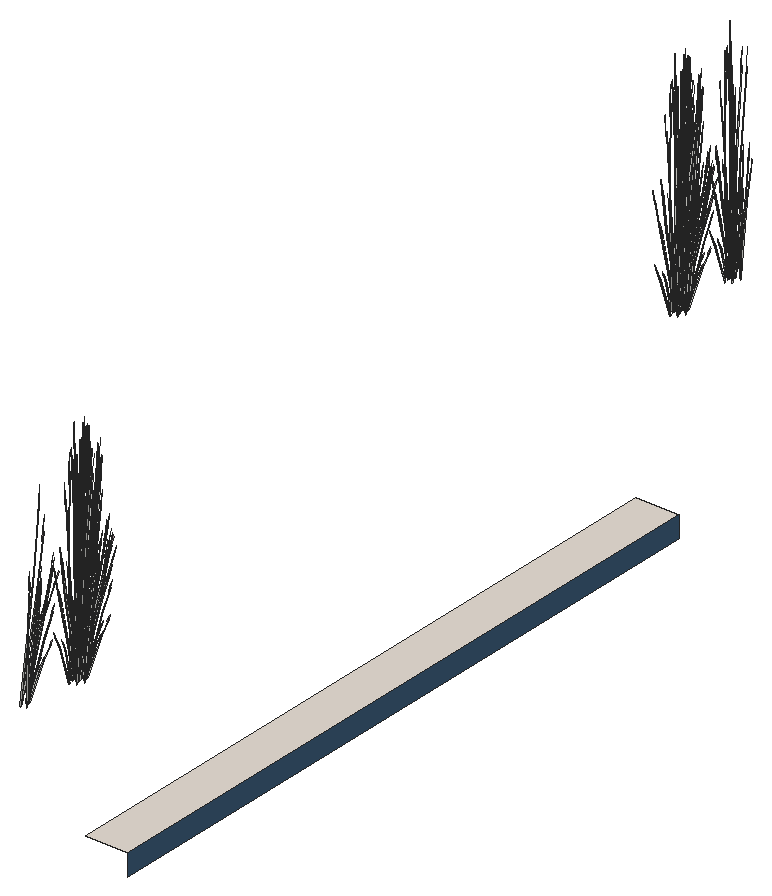
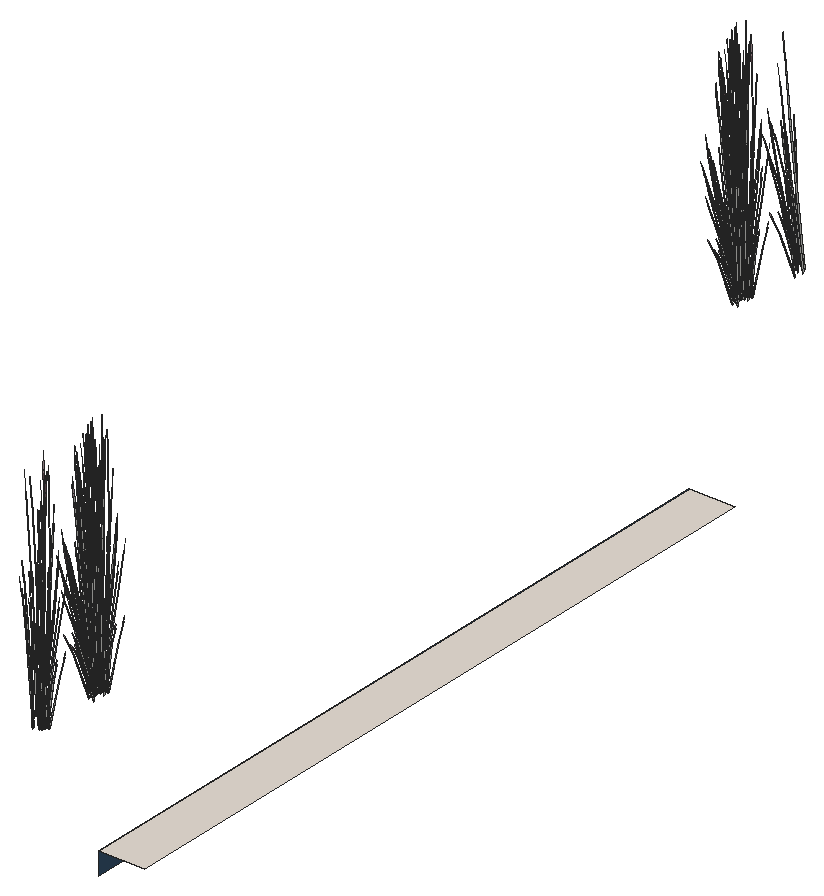
# SketchUp Ruby script. Lengths in inches.
U = 1.inch
M = Sketchup.active_model
def pt(a) = Geom::Point3d.new(a.map { |v| v * U })
def face(e, loops, mat)
  f = e.add_face(loops[0].map { |a| pt(a) })
  loops[1..].each { |l| e.add_face(l.map { |a| pt(a) }).erase! }
  f.material = f.back_material = mat if mat
  f
end
# faces: each face lists its corners as indices into pts; further lists are holes
def faces(e, pts, list, mat = nil) = list.each { |f| face(e, (f[0].is_a?(Array) ? f : [f]).map { |l| l.map { |i| pts[i] } }, mat) }
# xy, xz, yz: faces in a plane at the given z, y or x. An outline is a flat list of corners, or four numbers for a rectangle; further outlines are holes
def ring(l) = l.size == 4 ? [[l[0], l[1]], [l[2], l[1]], [l[2], l[3]], [l[0], l[3]]] : l.each_slice(2).to_a
def flat(e, list, mat, &to3) = list.each { |f| face(e, (f[0].is_a?(Array) ? f : [f]).map { |l| ring(l).map { |u, v| to3.(u, v) } }, mat) }
def xy(e, z, list, mat = nil) = flat(e, list, mat) { |x, y| [x, y, z] }
def xz(e, y, list, mat = nil) = flat(e, list, mat) { |x, z| [x, y, z] }
def yz(e, x, list, mat = nil) = flat(e, list, mat) { |y, z| [x, y, z] }
def lines(e, pts, list) = list.each { |a, b| e.add_line(pt(pts[a]), pt(pts[b])) }
# prism: a flat outline (further loops are holes) pulled along v
def prism(e, loops, v, mat = nil)
  f = face(e, loops, mat); d = Geom::Vector3d.new(v.map { |x| x * U })
  f.pushpull(f.normal.samedirection?(d) ? d.length : -d.length)
end
def box(e, o, s, mat = nil) = prism(e, [[o, [o[0] + s[0], o[1], o[2]], [o[0] + s[0], o[1] + s[1], o[2]], [o[0], o[1] + s[1], o[2]]]], [0, 0, s[2]], mat)
def at(x, y, z, deg = 0) = Geom::Transformation.translation(pt([x, y, z])) * Geom::Transformation.rotation(ORIGIN, Z_AXIS, deg.degrees)
def axes(o, x, y, z) = Geom::Transformation.new([*x, 0, *y, 0, *z, 0, *pt(o).to_a, 1])
def part(name) = M.definitions.add(name)
# library, detail: a bought-in or finely detailed component or shape, given as its bounding box
def library(name, o, s) = part(name).tap { |d| box(d.entities, o, s) }
def detail(e, o, s) = box(e.add_group.entities, o, s)
def put(e, d, t, mat = nil) = e.add_instance(d, t).tap { |i| i.material = mat if mat }
def group(e, t, mat = nil) = e.add_group.tap { |g| g.transformation = t; g.material = mat if mat }.entities
root = M.entities
M.materials.add("Carpet_04_1K").color = [56, 85, 112]
M.materials.add("LightPink_Translucent").color = [144, 107, 117]
M.materials["LightPink_Translucent"].alpha = 0.75
M.materials.add("Marble_01_1K").color = [230, 221, 211]
c1 = part("blade")
p = [[2.15,0.21,22],[0,0.17,0],[0.09,0.45,0],[2.18,0.31,22],[2.29,0.31,22],[0.38,0.45,0],
  [2.48,0.24,33],[2.49,0.24,33],[2.48,0.22,33]]
faces(c1.entities,p,[[0,1,2,3],[4,5,2,3],[6,3,4,7],[8,0,3,6]])
c2 = part("seeds")
p = [[0.3,-0.1,1.38],[-0.01,-0.03,1.59],[-0.01,-0.03,0.03],[0.14,-0.07,-0.07],[0.29,-0.03,3],[0.15,0.01,3.11]]
faces(c2.entities,p,[[0,1,2,3],[1,0,4,5]],"LightPink_Translucent")
c3 = part("blade with seeds")
put(c3.entities,c1,at(0,0,0))
put(c3.entities,c2,axes([2.4,0.25,30.99],[1.5799,-0.05474,1.17369],[-0.12525,1.92788,0.29478],[-0.07173,-0.02425,1.56792]))
xy(root,-42,[[398.57,316.3,410.57,509.26]],"Marble_01_1K")
yz(root,410.57,[[316.3,-48,509.26,-42]],"Carpet_04_1K")
put(root,c3,axes([400.96,292.9,1.98],[-0.22732,0.05597,1.41583],[-0.03618,-0.44548,0.08104],[0.15921,-0.06743,0.80566]))
put(root,c3,axes([401.37,292.51,2.26],[-0.21881,-0.29821,-0.06488],[0.23965,-0.27324,-0.29416],[0.0679,-0.01924,0.97024]))
put(root,c3,axes([400.54,292.9375,4.98],[0.31014,-0.20596,-0.71045],[0.17284,0.42397,0.08574],[0.14985,-0.04816,1.00501]))
put(root,c3,axes([401.2,292.61,1.49],[-0.01845,-0.0708,1.76342],[0.12793,-0.41416,-0.26939],[0.12905,-0.00596,0.30037]))
put(root,c3,axes([400.81,292.98,4.53],[0.29332,0.1301,-0.35414],[-0.08555,0.37955,0.4572],[0.11809,-0.0348,0.87481]))
put(root,c3,axes([400.29,291.34,2.02],[0.33032,0.23318,-0.49651],[-0.19744,0.41812,0],[0.07523,0.05311,1.57504]))
put(root,c3,axes([400.01,292.51,3.875],[-0.14639,0.01056,1.71376],[0.09712,-0.45778,0.13857],[0.20862,0.02831,0.73262]))
put(root,c3,axes([399.81,292.23,2.06],[0.36714,0.07646,-0.62353],[-0.07747,0.47163,-0.16365],[0.10956,0.05715,1.37633]))
put(root,c3,axes([401.43,293.06,2.77],[-0.21807,0.07699,1.1486],[0.10265,-0.31819,0.84392],[0.11568,0.02177,0.25299]))
put(root,c3,axes([401.05,294.04,3.93],[-0.06755,-0.39203,-0.03492],[0.31928,-0.09013,-0.15832],[0.06667,0.02485,0.52218]))
put(root,c3,axes([401.02,293.57,2.59],[-0.085,-0.1147,1.43002],[0.1106,-0.37943,-0.30754],[0.17198,0.0514,0.61141]))
put(root,c3,axes([400.24,293.8,4.98],[0.35281,0.01123,-0.71045],[-0.0237,0.47284,0.08574],[0.14947,0.0499,1.00501]))
put(root,c3,axes([400.45,293.99,4.53],[0.20082,0.29199,-0.35414],[-0.2293,0.2764,0.4572],[0.1165,0.04206,0.87481]))
put(root,c3,axes([399.73,293.24,3.875],[-0.1311,-0.08035,1.71376],[0.27131,-0.33708,0.13857],[0.16909,0.15206,0.73262]))
put(root,c3,axes([400.27,294.66,1.49],[0.02571,-0.06733,1.76342],[0.32373,-0.19829,-0.26939],[0.09815,0.10263,0.30037]))
put(root,c3,axes([399.77,294.34,4.68],[0.34827,-0.11086,-0.51099],[0.06092,0.41983,-0.3958],[0.09354,0.12031,0.97773]))
put(root,c3,axes([402.72,307.125,2.59],[-0.10032,0.0944,1.43002],[-0.30046,-0.16522,-0.30754],[0.05569,-0.20547,0.61141]))
put(root,c3,axes([401.98,306.61,1.49],[-0.0592,0.0168,1.76342],[-0.32738,-0.18913,-0.26939],[0.00549,-0.15776,0.30037]))
put(root,c3,axes([402.97,307.83,4.98],[0.00918,-0.43138,-0.71045],[0.38672,0.02897,0.08574],[0.04081,-0.18275,1.00501]))
put(root,c3,axes([402.3,307.13,4.53],[0.1064,-0.35863,-0.35414],[0.31043,0.1046,0.4572],[-0.02846,-0.14439,0.87481]))
put(root,c3,axes([402.53,307.61,3.875],[-0.06572,0.16029,1.71376],[-0.27569,-0.33172,0.13857],[0.12437,-0.20675,0.73262]))
put(root,c3,axes([402.35,306.375,2.77],[0.04528,0.27194,1.1486],[-0.25117,-0.15062,0.84392],[0.02703,-0.13924,0.25299]))
put(root,c3,axes([402.89,307.68,4.68],[-0.25266,-0.31335,-0.51099],[0.2669,-0.27442,-0.3958],[0.03844,-0.15921,0.97773]))
put(root,c3,axes([403.13,307.57,4.53],[0.23881,-0.24554,-0.35414],[0.22606,0.28036,0.4572],[0.0344,-0.14245,0.87481]))
put(root,c3,axes([403.43,307.42,1.49],[-0.05283,-0.03674,1.76342],[-0.13569,-0.41045,-0.26939],[0.09154,-0.11138,0.30037]))
put(root,c3,axes([403.42,308.57,4.98],[0.18436,-0.36797,-0.71045],[0.32306,0.26151,0.08574],[0.11008,-0.13332,1.00501]))
put(root,c3,axes([401.43,307.5,2.375],[-0.22066,-0.46731,0],[0.36918,-0.26061,-0.51607],[0.08408,-0.05936,1.63711]))
put(root,c3,axes([403.41,308.4,4.68],[-0.09067,-0.42583,-0.51099],[0.34336,-0.07449,-0.3958],[0.0984,-0.11438,0.97773]))
put(root,c3,axes([401.73,307.43,2.02],[0.33032,-0.23318,-0.49651],[0.19744,0.41812,0],[0.07523,-0.05311,1.57504]))
put(root,c3,axes([403.69,308.24,2.59],[-0.12609,-0.01381,1.43002],[-0.12917,-0.37055,-0.30754],[0.1549,-0.10482,0.61141]))
put(root,c3,axes([402.12,308.39,2.06],[0.23773,-0.35053,-0.62353],[0.29532,0.31785,-0.16365],[0.09526,-0.08744,1.37633]))
put(root,c3,axes([403.84,307.56,2.77],[-0.11756,0.2374,1.1486],[-0.10105,-0.31895,0.84392],[0.09709,-0.07992,0.25299]))
put(root,c3,axes([403.67,308.45,4.53],[0.30722,-0.06665,-0.35414],[0.08112,0.381,0.4572],[0.08804,-0.10234,0.87481]))
put(root,c3,axes([401.71,309,2.21],[0.17124,-0.42022,-0.44739],[0.35581,0.20224,0.21531],[0,-0.09687,1.43643]))
put(root,c3,axes([401.86,308.79,2.67],[-0.04113,-0.53214,-0.29095],[0.42835,-0.03218,-0.50002],[0.07543,-0.07088,1.59708]))
put(root,c3,axes([401.81,307.62,2.03],[0.32928,0.11539,-0.30978],[-0.08291,0.40636,0.30978],[0.06638,-0.04686,1.38974]))
put(root,c3,axes([401.92,309.21,2.43],[0.39767,0.22603,0.24065],[-0.19139,0.46966,0.50002],[0,-0.10827,1.60543]))
put(root,c3,axes([401.79,308.9,2.72],[-0.38326,0.02879,0.44739],[-0.03466,-0.47788,-0.21531],[0.06861,-0.04843,1.43643]))
put(root,c3,axes([403.57,309.35,4.68],[0.09562,-0.42421,-0.51099],[0.32782,0.1454,-0.3958],[0.13199,-0.0389,0.97773]))
put(root,c3,axes([403.06,307.62,2.375],[0.22066,-0.46731,0],[0.36918,0.26061,-0.51607],[0.08408,0.05936,1.63711]))
put(root,c3,axes([401.78,309.07,2.36],[0.15345,0.52148,0.45755],[-0.43845,0.18134,0.17955],[0.00536,-0.09582,1.58856]))
put(root,c3,axes([403.92,309.47,1.98],[-0.22732,0.05597,1.41583],[-0.03618,-0.44548,0.08104],[0.15921,-0.06743,0.80566]))
put(root,c3,axes([404.34,309.07,2.26],[-0.21881,-0.29821,-0.06488],[0.23965,-0.27324,-0.29416],[0.0679,-0.01924,0.97024]))
put(root,c3,axes([402.33,309.11,2.21],[0,-0.53961,0],[0.44133,0,0],[0,0,1.79456]))
put(root,c3,axes([402.87,307.87,2.48],[-0.33032,-0.23318,0.49651],[0.19744,-0.41812,0],[0.07523,0.05311,1.57504]))
put(root,c3,axes([403.51,309.5,4.98],[0.31014,-0.20596,-0.71045],[0.17284,0.42397,0.08574],[0.14985,-0.04816,1.00501]))
put(root,c3,axes([402.12,308.77,2.36],[-0.29264,0.42323,0.45755],[-0.34767,-0.3736,0.17955],[0.07055,-0.04224,1.58856]))
put(root,c3,axes([401.61,308.08,2.47],[-0.10196,0.46348,0.17642],[-0.3731,-0.13116,0.35086],[0.06445,-0.00226,1.60407]))
put(root,c3,axes([401.46,308.45,1.59],[-0.3474,0.18671,1.28929],[-0.11057,-0.53572,0.50096],[0.21332,0.00891,1.46642]))
put(root,c3,axes([402.39,308.59,2.62],[0.06809,-0.4162,0.1448],[0.33266,0.07225,-0.41347],[0.06054,0.04274,1.26744]))
put(root,c3,axes([404.17,309.18,1.49],[-0.01845,-0.0708,1.76342],[0.12793,-0.41416,-0.26939],[0.12905,-0.00596,0.30037]))
put(root,c3,axes([402.25,308.7,2.72],[-0.21202,-0.39143,0.44739],[0.32115,-0.27564,-0.21531],[0.06861,0.04843,1.43643]))
put(root,c3,axes([402.36,308.73,2.67],[0.35635,-0.30962,-0.29095],[0.23697,0.43749,-0.50002],[0.08792,0.04443,1.59708]))
put(root,c3,axes([403.78,309.54,4.53],[0.29332,0.1301,-0.35414],[-0.08555,0.37955,0.4572],[0.11809,-0.0348,0.87481]))
put(root,c3,axes([403.26,307.9,2.02],[0.33032,0.23318,-0.49651],[-0.19744,0.41812,0],[0.07523,0.05311,1.57504]))
put(root,c3,axes([402.63,309.23,2.21],[0.39487,0,0],[0,0.48281,0],[0,0,1.78407]))
put(root,c3,axes([402.74,308.1,2.47],[-0.37926,0.12378,0.17642],[-0.09365,-0.46065,0.35086],[0.03382,0.06712,1.60407]))
put(root,c3,axes([402.98,309.07,3.875],[-0.14639,0.01056,1.71376],[0.09712,-0.45778,0.13857],[0.20862,0.02831,0.73262]))
put(root,c3,axes([403.17,308.08,2.03],[0.08291,0.40636,-0.30978],[-0.32928,0.11539,0.30978],[0.06638,0.04686,1.38974]))
put(root,c3,axes([402.5,308.99,2.38],[-0.44609,-0.09826,0.49198],[0.09078,-0.55493,0.19306],[0.06519,0.05359,1.70813]))
put(root,c3,axes([402.15,310.36,2.2],[-0.11516,-0.40207,0],[0.32884,-0.1408,0],[0,0,1.54371]))
put(root,c3,axes([402.58,310.3,2.18],[0.37054,-0.15823,-0.19198],[0.1302,0.45581,0.00008],[0.0409,-0.01749,1.73897]))
put(root,c3,axes([402.62,309.44,2.21],[0.24637,0.30123,0],[-0.24637,0.30123,0],[0,0,1.69266]))
put(root,c3,axes([403.29,309.31,2.47],[-0.2773,-0.3397,0.17642],[0.27945,-0.32949,0.35086],[-0.03063,0.06937,1.60407]))
put(root,c3,axes([402.78,308.8,2.06],[0.36714,0.07646,-0.62353],[-0.07747,0.47163,-0.16365],[0.10956,0.05715,1.37633]))
put(root,c3,axes([404.4,309.62,2.77],[-0.21807,0.07699,1.1486],[0.10265,-0.31819,0.84392],[0.11568,0.02177,0.25299]))
put(root,c3,axes([402.62,309.09,2.72],[0.17124,-0.42022,0.44739],[0.35581,0.20224,-0.21531],[0,0.09687,1.43643]))
put(root,c3,axes([402.55,309.33,2.29],[0,0.53934,-0.05637],[-0.44133,0,0],[0,0.01695,1.79368]))
put(root,c3,axes([402.58,308.95,2.21],[0.21202,0.39143,-0.44739],[-0.32115,0.27564,0.21531],[0.06861,0.04843,1.43643]))
put(root,c3,axes([404.02,310.6,3.93],[-0.06755,-0.39203,-0.03492],[0.31928,-0.09013,-0.15832],[0.06667,0.02485,0.52218]))
put(root,c3,axes([403.52,309.32,2.48],[0,-0.46636,0.49651],[0.39487,0,0],[0,0.10622,1.57504]))
put(root,c3,axes([402.77,309.18,2.62],[0.32884,-0.136,0.1448],[0.11516,0.38837,-0.41347],[0,0.08547,1.26744]))
put(root,c3,axes([403.99,310.13,2.59],[-0.085,-0.1147,1.43002],[0.1106,-0.37943,-0.30754],[0.17198,0.0514,0.61141]))
put(root,c3,axes([402.47,310.55,2.2],[0.35581,0.20937,0],[-0.17124,0.43505,0],[0,0,1.74954]))
put(root,c3,axes([403.21,310.36,4.98],[0.35281,0.01123,-0.71045],[-0.0237,0.47284,0.08574],[0.14947,0.0499,1.00501]))
put(root,c3,axes([402.8125,310.74,2.48],[0.33032,-0.23318,0.49651],[0.19744,0.41812,0],[-0.07523,0.05311,1.57504]))
put(root,c3,axes([402.34,310.37,2.29],[0.15345,0.53576,-0.06012],[-0.43845,0.18773,0],[0.00536,0.01871,1.72173]))
put(root,c3,axes([403.78,309.4,2.375],[0.44133,0,0],[0,0.52122,-0.51607],[0,0.11871,1.63711]))
put(root,c3,axes([403.61,309.67,2.2],[-0.44111,-0.00373,-0.04976],[0,-0.52122,0.49943],[-0.01386,0.11865,1.58352]))
put(root,c3,axes([402.65,309.22,2.67],[0.39748,0.22252,-0.29095],[-0.19139,0.46966,-0.50002],[0.01249,0.11531,1.59708]))
put(root,c3,axes([403.42,310.56,4.53],[0.20082,0.29199,-0.35414],[-0.2293,0.2764,0.4572],[0.1165,0.04206,0.87481]))
put(root,c3,axes([403.52,309.74,2.03],[-0.24637,0.29097,-0.30978],[-0.24637,-0.29097,0.30978],[0,0.09372,1.38974]))
put(root,c3,axes([402.61,309.5625,2.21],[-0.17124,0.42022,-0.44739],[-0.35581,-0.20224,0.21531],[0,0.09687,1.43643]))
put(root,c3,axes([402.62,310.77,2.33],[0.44186,0.15158,0.30756],[-0.11054,0.54181,-0.36492],[-0.07313,0.06781,1.64885]))
put(root,c3,axes([403.6875,309.75,2.02],[0,0.46636,-0.49651],[-0.39487,0,0],[0,0.10622,1.57504]))
put(root,c3,axes([402.7,309.81,3.875],[-0.1311,-0.08035,1.71376],[0.27131,-0.33708,0.13857],[0.16909,0.15206,0.73262]))
put(root,c3,axes([403.18,310.72,2.77],[-0.19872,-0.13409,1.1486],[0.2566,-0.13625,0.84392],[0.06921,0.11541,0.25299]))
put(root,c3,axes([403.24,311.22,1.49],[0.02571,-0.06733,1.76342],[0.32373,-0.19829,-0.26939],[0.09815,0.10263,0.30037]))
put(root,c3,axes([402.8125,309.69,2.09],[0.12941,0.42699,-0.69212],[-0.37279,0.15378,-0.18165],[0.0143,0.14459,1.52773]))
put(root,c3,axes([402.74,310.91,4.68],[0.34827,-0.11086,-0.51099],[0.06092,0.41983,-0.3958],[0.09354,0.12031,0.97773]))
put(root,c3,axes([403.22,311.33,2.67],[-0.22633,-0.01463,1.0506],[0.14947,-0.31064,0.58006],[0.08941,0.11036,0.8241]))
put(root,c3,axes([402.48,310.58,2.59],[0.00623,-0.15459,1.43002],[0.29764,-0.17268,-0.30754],[0.09188,0.18503,0.61141]))
put(root,c3,axes([401.73,311.21,1.49],[0.05712,-0.02538,1.76342],[0.34359,0.13968,-0.26939],[0.01005,0.15742,0.30037]))
put(root,c3,axes([401.96,311.1,4.68],[0.34695,0.11691,-0.51099],[-0.11892,0.40083,-0.3958],[0.03181,0.16138,0.97773]))
put(root,c3,axes([402.16,310.27,3.875],[-0.08068,-0.14973,1.71376],[0.3728,-0.12606,0.13857],[0.08426,0.23506,0.73262]))
put(root,c3,axes([401.8,311.35,4.53],[-0.1064,0.35863,-0.35414],[-0.31043,-0.1046,0.4572],[0.02846,0.14439,0.87481]))
put(root,c3,axes([401.84,311.03,4.98],[0.16845,0.3792,-0.71045],[-0.34676,0.21133,0.08574],[0.03939,0.18322,1.00501]))
put(root,c3,axes([402.72,517.5625,2.59],[-0.10032,0.0944,1.43002],[-0.30046,-0.16522,-0.30754],[0.05569,-0.20547,0.61141]))
put(root,c3,axes([401.98,517.05,1.49],[-0.0592,0.0168,1.76342],[-0.32738,-0.18913,-0.26939],[0.00549,-0.15776,0.30037]))
put(root,c3,axes([402.97,518.26,4.98],[0.00918,-0.43138,-0.71045],[0.38672,0.02897,0.08574],[0.04081,-0.18275,1.00501]))
put(root,c3,axes([402.3,517.57,4.53],[0.1064,-0.35863,-0.35414],[0.31043,0.1046,0.4572],[-0.02846,-0.14439,0.87481]))
put(root,c3,axes([402.53,518.04,3.875],[-0.06572,0.16029,1.71376],[-0.27569,-0.33172,0.13857],[0.12437,-0.20675,0.73262]))
put(root,c3,axes([402.35,516.81,2.77],[0.04528,0.27194,1.1486],[-0.25117,-0.15062,0.84392],[0.02703,-0.13924,0.25299]))
put(root,c3,axes([402.89,518.12,4.68],[-0.25266,-0.31335,-0.51099],[0.2669,-0.27442,-0.3958],[0.03844,-0.15921,0.97773]))
put(root,c3,axes([403.13,518,4.53],[0.23881,-0.24554,-0.35414],[0.22606,0.28036,0.4572],[0.0344,-0.14245,0.87481]))
put(root,c3,axes([403.43,517.85,1.49],[-0.05283,-0.03674,1.76342],[-0.13569,-0.41045,-0.26939],[0.09154,-0.11138,0.30037]))
put(root,c3,axes([403.42,519.01,4.98],[0.18436,-0.36797,-0.71045],[0.32306,0.26151,0.08574],[0.11008,-0.13332,1.00501]))
put(root,c3,axes([401.43,517.9375,2.375],[-0.22066,-0.46731,0],[0.36918,-0.26061,-0.51607],[0.08408,-0.05936,1.63711]))
put(root,c3,axes([403.41,518.84,4.68],[-0.09067,-0.42583,-0.51099],[0.34336,-0.07449,-0.3958],[0.0984,-0.11438,0.97773]))
put(root,c3,axes([401.73,517.87,2.02],[0.33032,-0.23318,-0.49651],[0.19744,0.41812,0],[0.07523,-0.05311,1.57504]))
put(root,c3,axes([403.69,518.67,2.59],[-0.12609,-0.01381,1.43002],[-0.12917,-0.37055,-0.30754],[0.1549,-0.10482,0.61141]))
put(root,c3,axes([402.12,518.82,2.06],[0.23773,-0.35053,-0.62353],[0.29532,0.31785,-0.16365],[0.09526,-0.08744,1.37633]))
put(root,c3,axes([403.84,517.99,2.77],[-0.11756,0.2374,1.1486],[-0.10105,-0.31895,0.84392],[0.09709,-0.07992,0.25299]))
put(root,c3,axes([403.67,518.88,4.53],[0.30722,-0.06665,-0.35414],[0.08112,0.381,0.4572],[0.08804,-0.10234,0.87481]))
put(root,c3,axes([401.71,519.4375,2.21],[0.17124,-0.42022,-0.44739],[0.35581,0.20224,0.21531],[0,-0.09687,1.43643]))
put(root,c3,axes([401.86,519.23,2.67],[-0.04113,-0.53214,-0.29095],[0.42835,-0.03218,-0.50002],[0.07543,-0.07088,1.59708]))
put(root,c3,axes([401.81,518.05,2.03],[0.32928,0.11539,-0.30978],[-0.08291,0.40636,0.30978],[0.06638,-0.04686,1.38974]))
put(root,c3,axes([401.92,519.65,2.43],[0.39767,0.22603,0.24065],[-0.19139,0.46966,0.50002],[0,-0.10827,1.60543]))
put(root,c3,axes([401.79,519.33,2.72],[-0.38326,0.02879,0.44739],[-0.03466,-0.47788,-0.21531],[0.06861,-0.04843,1.43643]))
put(root,c3,axes([403.57,519.78,4.68],[0.09562,-0.42421,-0.51099],[0.32782,0.1454,-0.3958],[0.13199,-0.0389,0.97773]))
put(root,c3,axes([403.06,518.06,2.375],[0.22066,-0.46731,0],[0.36918,0.26061,-0.51607],[0.08408,0.05936,1.63711]))
put(root,c3,axes([401.78,519.5,2.36],[0.15345,0.52148,0.45755],[-0.43845,0.18134,0.17955],[0.00536,-0.09582,1.58856]))
put(root,c3,axes([403.92,519.9,1.98],[-0.22732,0.05597,1.41583],[-0.03618,-0.44548,0.08104],[0.15921,-0.06743,0.80566]))
put(root,c3,axes([404.34,519.51,2.26],[-0.21881,-0.29821,-0.06488],[0.23965,-0.27324,-0.29416],[0.0679,-0.01924,0.97024]))
put(root,c3,axes([402.33,519.55,2.21],[0,-0.53961,0],[0.44133,0,0],[0,0,1.79456]))
put(root,c3,axes([402.87,518.3,2.48],[-0.33032,-0.23318,0.49651],[0.19744,-0.41812,0],[0.07523,0.05311,1.57504]))
put(root,c3,axes([403.51,519.9375,4.98],[0.31014,-0.20596,-0.71045],[0.17284,0.42397,0.08574],[0.14985,-0.04816,1.00501]))
put(root,c3,axes([402.12,519.21,2.36],[-0.29264,0.42323,0.45755],[-0.34767,-0.3736,0.17955],[0.07055,-0.04224,1.58856]))
put(root,c3,axes([401.61,518.51,2.47],[-0.10196,0.46348,0.17642],[-0.3731,-0.13116,0.35086],[0.06445,-0.00226,1.60407]))
put(root,c3,axes([401.46,518.89,1.59],[-0.3474,0.18671,1.28929],[-0.11057,-0.53572,0.50096],[0.21332,0.00891,1.46642]))
put(root,c3,axes([402.39,519.03,2.62],[0.06809,-0.4162,0.1448],[0.33266,0.07225,-0.41347],[0.06054,0.04274,1.26744]))
put(root,c3,axes([404.17,519.61,1.49],[-0.01845,-0.0708,1.76342],[0.12793,-0.41416,-0.26939],[0.12905,-0.00596,0.30037]))
put(root,c3,axes([402.25,519.14,2.72],[-0.21202,-0.39143,0.44739],[0.32115,-0.27564,-0.21531],[0.06861,0.04843,1.43643]))
put(root,c3,axes([402.36,519.16,2.67],[0.35635,-0.30962,-0.29095],[0.23697,0.43749,-0.50002],[0.08792,0.04443,1.59708]))
put(root,c3,axes([403.78,519.98,4.53],[0.29332,0.1301,-0.35414],[-0.08555,0.37955,0.4572],[0.11809,-0.0348,0.87481]))
put(root,c3,axes([403.26,518.34,2.02],[0.33032,0.23318,-0.49651],[-0.19744,0.41812,0],[0.07523,0.05311,1.57504]))
put(root,c3,axes([402.63,519.67,2.21],[0.39487,0,0],[0,0.48281,0],[0,0,1.78407]))
put(root,c3,axes([402.74,518.54,2.47],[-0.37926,0.12378,0.17642],[-0.09365,-0.46065,0.35086],[0.03382,0.06712,1.60407]))
put(root,c3,axes([402.98,519.51,3.875],[-0.14639,0.01056,1.71376],[0.09712,-0.45778,0.13857],[0.20862,0.02831,0.73262]))
put(root,c3,axes([403.17,518.51,2.03],[0.08291,0.40636,-0.30978],[-0.32928,0.11539,0.30978],[0.06638,0.04686,1.38974]))
put(root,c3,axes([402.5,519.42,2.38],[-0.44609,-0.09826,0.49198],[0.09078,-0.55493,0.19306],[0.06519,0.05359,1.70813]))
put(root,c3,axes([402.15,520.79,2.2],[-0.11516,-0.40207,0],[0.32884,-0.1408,0],[0,0,1.54371]))
put(root,c3,axes([402.58,520.74,2.18],[0.37054,-0.15823,-0.19198],[0.1302,0.45581,0.00008],[0.0409,-0.01749,1.73897]))
put(root,c3,axes([402.62,519.875,2.21],[0.24637,0.30123,0],[-0.24637,0.30123,0],[0,0,1.69266]))
put(root,c3,axes([403.29,519.74,2.47],[-0.2773,-0.3397,0.17642],[0.27945,-0.32949,0.35086],[-0.03063,0.06937,1.60407]))
put(root,c3,axes([402.78,519.23,2.06],[0.36714,0.07646,-0.62353],[-0.07747,0.47163,-0.16365],[0.10956,0.05715,1.37633]))
put(root,c3,axes([404.4,520.06,2.77],[-0.21807,0.07699,1.1486],[0.10265,-0.31819,0.84392],[0.11568,0.02177,0.25299]))
put(root,c3,axes([402.62,519.52,2.72],[0.17124,-0.42022,0.44739],[0.35581,0.20224,-0.21531],[0,0.09687,1.43643]))
put(root,c3,axes([402.55,519.76,2.29],[0,0.53934,-0.05637],[-0.44133,0,0],[0,0.01695,1.79368]))
put(root,c3,axes([402.58,519.38,2.21],[0.21202,0.39143,-0.44739],[-0.32115,0.27564,0.21531],[0.06861,0.04843,1.43643]))
put(root,c3,axes([404.02,521.04,3.93],[-0.06755,-0.39203,-0.03492],[0.31928,-0.09013,-0.15832],[0.06667,0.02485,0.52218]))
put(root,c3,axes([403.52,519.76,2.48],[0,-0.46636,0.49651],[0.39487,0,0],[0,0.10622,1.57504]))
put(root,c3,axes([402.77,519.62,2.62],[0.32884,-0.136,0.1448],[0.11516,0.38837,-0.41347],[0,0.08547,1.26744]))
put(root,c3,axes([403.99,520.57,2.59],[-0.085,-0.1147,1.43002],[0.1106,-0.37943,-0.30754],[0.17198,0.0514,0.61141]))
put(root,c3,axes([402.47,520.98,2.2],[0.35581,0.20937,0],[-0.17124,0.43505,0],[0,0,1.74954]))
put(root,c3,axes([403.21,520.8,4.98],[0.35281,0.01123,-0.71045],[-0.0237,0.47284,0.08574],[0.14947,0.0499,1.00501]))
put(root,c3,axes([402.8125,521.18,2.48],[0.33032,-0.23318,0.49651],[0.19744,0.41812,0],[-0.07523,0.05311,1.57504]))
put(root,c3,axes([402.34,520.81,2.29],[0.15345,0.53576,-0.06012],[-0.43845,0.18773,0],[0.00536,0.01871,1.72173]))
put(root,c3,axes([403.78,519.84,2.375],[0.44133,0,0],[0,0.52122,-0.51607],[0,0.11871,1.63711]))
put(root,c3,axes([403.61,520.1,2.2],[-0.44111,-0.00373,-0.04976],[0,-0.52122,0.49943],[-0.01386,0.11865,1.58352]))
put(root,c3,axes([402.65,519.65,2.67],[0.39748,0.22252,-0.29095],[-0.19139,0.46966,-0.50002],[0.01249,0.11531,1.59708]))
put(root,c3,axes([403.42,520.99,4.53],[0.20082,0.29199,-0.35414],[-0.2293,0.2764,0.4572],[0.1165,0.04206,0.87481]))
put(root,c3,axes([403.52,520.18,2.03],[-0.24637,0.29097,-0.30978],[-0.24637,-0.29097,0.30978],[0,0.09372,1.38974]))
put(root,c3,axes([402.61,520,2.21],[-0.17124,0.42022,-0.44739],[-0.35581,-0.20224,0.21531],[0,0.09687,1.43643]))
put(root,c3,axes([402.62,521.21,2.33],[0.44186,0.15158,0.30756],[-0.11054,0.54181,-0.36492],[-0.07313,0.06781,1.64885]))
put(root,c3,axes([403.6875,520.19,2.02],[0,0.46636,-0.49651],[-0.39487,0,0],[0,0.10622,1.57504]))
put(root,c3,axes([402.7,520.24,3.875],[-0.1311,-0.08035,1.71376],[0.27131,-0.33708,0.13857],[0.16909,0.15206,0.73262]))
put(root,c3,axes([403.18,521.16,2.77],[-0.19872,-0.13409,1.1486],[0.2566,-0.13625,0.84392],[0.06921,0.11541,0.25299]))
put(root,c3,axes([403.24,521.66,1.49],[0.02571,-0.06733,1.76342],[0.32373,-0.19829,-0.26939],[0.09815,0.10263,0.30037]))
put(root,c3,axes([402.8125,520.125,2.09],[0.12941,0.42699,-0.69212],[-0.37279,0.15378,-0.18165],[0.0143,0.14459,1.52773]))
put(root,c3,axes([402.74,521.34,4.68],[0.34827,-0.11086,-0.51099],[0.06092,0.41983,-0.3958],[0.09354,0.12031,0.97773]))
put(root,c3,axes([403.22,521.77,2.67],[-0.22633,-0.01463,1.0506],[0.14947,-0.31064,0.58006],[0.08941,0.11036,0.8241]))
put(root,c3,axes([402.48,521.01,2.59],[0.00623,-0.15459,1.43002],[0.29764,-0.17268,-0.30754],[0.09188,0.18503,0.61141]))
put(root,c3,axes([401.73,521.64,1.49],[0.05712,-0.02538,1.76342],[0.34359,0.13968,-0.26939],[0.01005,0.15742,0.30037]))
put(root,c3,axes([401.96,521.54,4.68],[0.34695,0.11691,-0.51099],[-0.11892,0.40083,-0.3958],[0.03181,0.16138,0.97773]))
put(root,c3,axes([402.16,520.71,3.875],[-0.08068,-0.14973,1.71376],[0.3728,-0.12606,0.13857],[0.08426,0.23506,0.73262]))
put(root,c3,axes([401.8,521.78,4.53],[-0.1064,0.35863,-0.35414],[-0.31043,-0.1046,0.4572],[0.02846,0.14439,0.87481]))
put(root,c3,axes([401.84,521.46,4.98],[0.16845,0.3792,-0.71045],[-0.34676,0.21133,0.08574],[0.03939,0.18322,1.00501]))
put(root,c3,axes([402.72,536.79,2.59],[-0.10032,0.0944,1.43002],[-0.30046,-0.16522,-0.30754],[0.05569,-0.20547,0.61141]))
put(root,c3,axes([401.98,536.28,1.49],[-0.0592,0.0168,1.76342],[-0.32738,-0.18913,-0.26939],[0.00549,-0.15776,0.30037]))
put(root,c3,axes([402.97,537.49,4.98],[0.00918,-0.43138,-0.71045],[0.38672,0.02897,0.08574],[0.04081,-0.18275,1.00501]))
put(root,c3,axes([402.3,536.8,4.53],[0.1064,-0.35863,-0.35414],[0.31043,0.1046,0.4572],[-0.02846,-0.14439,0.87481]))
put(root,c3,axes([402.53,537.27,3.875],[-0.06572,0.16029,1.71376],[-0.27569,-0.33172,0.13857],[0.12437,-0.20675,0.73262]))
put(root,c3,axes([402.35,536.04,2.77],[0.04528,0.27194,1.1486],[-0.25117,-0.15062,0.84392],[0.02703,-0.13924,0.25299]))
put(root,c3,axes([402.89,537.35,4.68],[-0.25266,-0.31335,-0.51099],[0.2669,-0.27442,-0.3958],[0.03844,-0.15921,0.97773]))
put(root,c3,axes([403.13,537.23,4.53],[0.23881,-0.24554,-0.35414],[0.22606,0.28036,0.4572],[0.0344,-0.14245,0.87481]))
put(root,c3,axes([403.43,537.08,1.49],[-0.05283,-0.03674,1.76342],[-0.13569,-0.41045,-0.26939],[0.09154,-0.11138,0.30037]))
put(root,c3,axes([403.42,538.24,4.98],[0.18436,-0.36797,-0.71045],[0.32306,0.26151,0.08574],[0.11008,-0.13332,1.00501]))
put(root,c3,axes([401.43,537.17,2.375],[-0.22066,-0.46731,0],[0.36918,-0.26061,-0.51607],[0.08408,-0.05936,1.63711]))
put(root,c3,axes([403.41,538.07,4.68],[-0.09067,-0.42583,-0.51099],[0.34336,-0.07449,-0.3958],[0.0984,-0.11438,0.97773]))
put(root,c3,axes([401.73,537.1,2.02],[0.33032,-0.23318,-0.49651],[0.19744,0.41812,0],[0.07523,-0.05311,1.57504]))
put(root,c3,axes([403.69,537.9,2.59],[-0.12609,-0.01381,1.43002],[-0.12917,-0.37055,-0.30754],[0.1549,-0.10482,0.61141]))
put(root,c3,axes([402.12,538.05,2.06],[0.23773,-0.35053,-0.62353],[0.29532,0.31785,-0.16365],[0.09526,-0.08744,1.37633]))
put(root,c3,axes([403.84,537.22,2.77],[-0.11756,0.2374,1.1486],[-0.10105,-0.31895,0.84392],[0.09709,-0.07992,0.25299]))
put(root,c3,axes([403.67,538.11,4.53],[0.30722,-0.06665,-0.35414],[0.08112,0.381,0.4572],[0.08804,-0.10234,0.87481]))
put(root,c3,axes([401.71,538.67,2.21],[0.17124,-0.42022,-0.44739],[0.35581,0.20224,0.21531],[0,-0.09687,1.43643]))
put(root,c3,axes([401.86,538.46,2.67],[-0.04113,-0.53214,-0.29095],[0.42835,-0.03218,-0.50002],[0.07543,-0.07088,1.59708]))
put(root,c3,axes([401.81,537.28,2.03],[0.32928,0.11539,-0.30978],[-0.08291,0.40636,0.30978],[0.06638,-0.04686,1.38974]))
put(root,c3,axes([401.92,538.875,2.43],[0.39767,0.22603,0.24065],[-0.19139,0.46966,0.50002],[0,-0.10827,1.60543]))
put(root,c3,axes([401.79,538.56,2.72],[-0.38326,0.02879,0.44739],[-0.03466,-0.47788,-0.21531],[0.06861,-0.04843,1.43643]))
put(root,c3,axes([403.57,539.01,4.68],[0.09562,-0.42421,-0.51099],[0.32782,0.1454,-0.3958],[0.13199,-0.0389,0.97773]))
put(root,c3,axes([403.06,537.29,2.375],[0.22066,-0.46731,0],[0.36918,0.26061,-0.51607],[0.08408,0.05936,1.63711]))
put(root,c3,axes([401.78,538.73,2.36],[0.15345,0.52148,0.45755],[-0.43845,0.18134,0.17955],[0.00536,-0.09582,1.58856]))
put(root,c3,axes([403.92,539.13,1.98],[-0.22732,0.05597,1.41583],[-0.03618,-0.44548,0.08104],[0.15921,-0.06743,0.80566]))
put(root,c3,axes([404.34,538.74,2.26],[-0.21881,-0.29821,-0.06488],[0.23965,-0.27324,-0.29416],[0.0679,-0.01924,0.97024]))
put(root,c3,axes([402.33,538.78,2.21],[0,-0.53961,0],[0.44133,0,0],[0,0,1.79456]))
put(root,c3,axes([402.87,537.53,2.48],[-0.33032,-0.23318,0.49651],[0.19744,-0.41812,0],[0.07523,0.05311,1.57504]))
